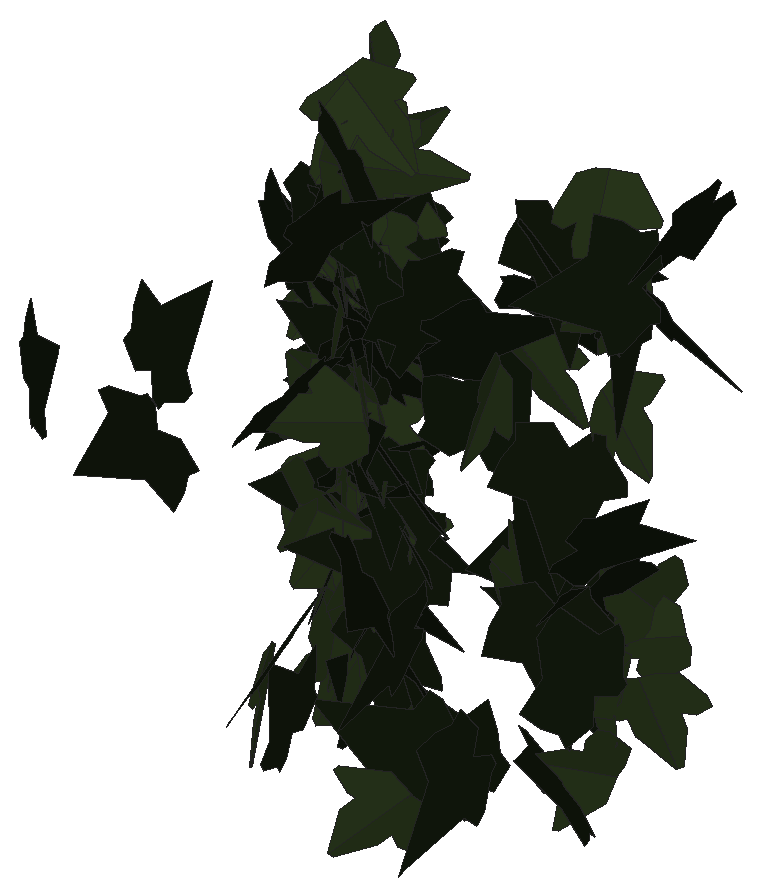
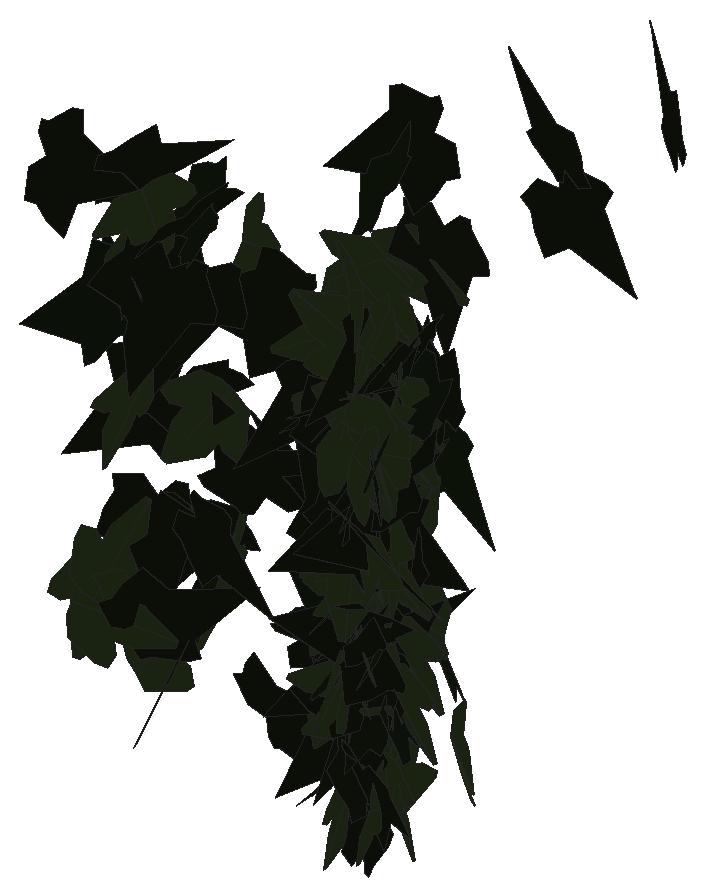
# SketchUp Ruby script. Lengths in inches.
U = 1.inch
M = Sketchup.active_model
def pt(a) = Geom::Point3d.new(a.map { |v| v * U })
def face(e, loops, mat)
  f = e.add_face(loops[0].map { |a| pt(a) })
  loops[1..].each { |l| e.add_face(l.map { |a| pt(a) }).erase! }
  f.material = f.back_material = mat if mat
  f
end
# faces: each face lists its corners as indices into pts; further lists are holes
def faces(e, pts, list, mat = nil) = list.each { |f| face(e, (f[0].is_a?(Array) ? f : [f]).map { |l| l.map { |i| pts[i] } }, mat) }
# xy, xz, yz: faces in a plane at the given z, y or x. An outline is a flat list of corners, or four numbers for a rectangle; further outlines are holes
def ring(l) = l.size == 4 ? [[l[0], l[1]], [l[2], l[1]], [l[2], l[3]], [l[0], l[3]]] : l.each_slice(2).to_a
def flat(e, list, mat, &to3) = list.each { |f| face(e, (f[0].is_a?(Array) ? f : [f]).map { |l| ring(l).map { |u, v| to3.(u, v) } }, mat) }
def xy(e, z, list, mat = nil) = flat(e, list, mat) { |x, y| [x, y, z] }
def xz(e, y, list, mat = nil) = flat(e, list, mat) { |x, z| [x, y, z] }
def yz(e, x, list, mat = nil) = flat(e, list, mat) { |y, z| [x, y, z] }
def lines(e, pts, list) = list.each { |a, b| e.add_line(pt(pts[a]), pt(pts[b])) }
# prism: a flat outline (further loops are holes) pulled along v
def prism(e, loops, v, mat = nil)
  f = face(e, loops, mat); d = Geom::Vector3d.new(v.map { |x| x * U })
  f.pushpull(f.normal.samedirection?(d) ? d.length : -d.length)
end
def box(e, o, s, mat = nil) = prism(e, [[o, [o[0] + s[0], o[1], o[2]], [o[0] + s[0], o[1] + s[1], o[2]], [o[0], o[1] + s[1], o[2]]]], [0, 0, s[2]], mat)
def at(x, y, z, deg = 0) = Geom::Transformation.translation(pt([x, y, z])) * Geom::Transformation.rotation(ORIGIN, Z_AXIS, deg.degrees)
def axes(o, x, y, z) = Geom::Transformation.new([*x, 0, *y, 0, *z, 0, *pt(o).to_a, 1])
def part(name) = M.definitions.add(name)
# library, detail: a bought-in or finely detailed component or shape, given as its bounding box
def library(name, o, s) = part(name).tap { |d| box(d.entities, o, s) }
def detail(e, o, s) = box(e.add_group.entities, o, s)
def put(e, d, t, mat = nil) = e.add_instance(d, t).tap { |i| i.material = mat if mat }
def group(e, t, mat = nil) = e.add_group.tap { |g| g.transformation = t; g.material = mat if mat }.entities
root = M.entities
M.materials.add("efeu1").color = [18, 25, 13]
M.materials.add("efeu2").color = [43, 57, 29]
c1 = part("ivyleaf_10")
p = [[0,0.5,-0.03],[-0.0625,2.02,-0.43],[-0.19,2.01,-0.46],[-0.54,1.05,-0.29],[-0.52,0.625,-0.18],[-0.83,0.76,-0.28],
  [-1.16,0.64,-0.33],[-1.15,0.33,-0.24],[-0.77,-0.39,0.02],[-0.3,-0.51,0.16],[0.04,-0.48,0.23],[-0.02,2.01,-0.4375],
  [-0.06,2.01,-0.43],[0.04,-0.49,0.23],[0.67,-0.49,0.14],[1.38,0.36,-0.2],[1.375,0.51,-0.24],[0.81,0.65,-0.19],
  [0.62,0.59,-0.15],[0.6,1.09,-0.28],[0.5,1.23,-0.31]]
faces(c1.entities,p,[[0,1,2,3,4,5,6,7,8,9,10],[11,12,0,13,14,15,16,17,18,19,20]],"efeu2")
c2 = part("ivyleaf_9")
p = [[1.54,2.16,1.25],[1.36,2.04,1.19],[-0.21,0.99,0.68],[-0.71,1.11,0.82],[-0.85,0.86,0.67],[-0.8,0.17,0.21],
  [-0.9,-0.01,0.1],[-0.67,-0.16,-0.02],[-0.08,-0.08,-0.05],[-0.03,-0.6,-0.4],[0.65,-0.88,-0.66],[0.83,-0.6,-0.49],
  [1.29,-0.42,-0.43],[1.8125,-0.07,-0.26],[1.21,0.44,0.15]]
faces(c2.entities,p,[[0,1,2,3,4,5,6,7,8,9,10,11,12,13,14]],"efeu1")
put(root,c1,axes([46.83,221.1,208.74],[0.39164,-0.18559,-0.24935],[-0.22582,0.10576,-0.43338],[0.2136,0.45208,-0.00098]))
put(root,c1,axes([46.84,221.05,209.32],[0.42383,-0.11987,-0.23664],[-0.22766,0.06455,-0.44046],[0.13615,0.48111,0.00014]))
put(root,c1,axes([46.65,221.74,207.45],[-0.01343,0.23322,-0.44207],[0.03841,-0.44044,-0.23353],[-0.49834,-0.04023,-0.00609]))
put(root,c2,axes([46.47,220.7,212.16],[-0.01841,0.02309,0.49913],[0.23908,-0.43817,0.02909],[0.43875,0.23974,0.00509]))
put(root,c1,axes([46.95,221.2,210.63],[-0.43209,0.10694,0.22774],[-0.22152,0.05288,-0.44512],[-0.11929,-0.48556,0.00168]))
put(root,c1,axes([46.85,221.12,210.37],[-0.18313,-0.32588,-0.33206],[-0.16064,-0.29062,0.37381],[-0.43664,0.2436,0.00175]))
put(root,c2,axes([46.55,221.15,212.125],[0.41245,-0.22857,-0.16625],[0.14512,-0.08112,0.47155],[-0.24254,-0.43723,-0.00058]))
put(root,c2,axes([46.96,221.4,209.11],[-0.12755,-0.05771,0.48],[-0.33346,-0.34894,-0.13056],[0.35006,-0.35342,0.05052]))
put(root,c2,axes([47.17,221.42,210.67],[-0.37965,0.24229,0.21716],[-0.1893,0.10694,-0.45025],[-0.26464,-0.4241,0.01053]))
put(root,c2,axes([46.76,221.76,207.88],[-0.37467,-0.03207,-0.32954],[0.32765,0.03568,-0.376],[0.04763,-0.49769,-0.00572]))
put(root,c1,axes([47.1,221.13,210.36],[0.25748,-0.10183,-0.41633],[-0.38457,0.15956,-0.27686],[0.18924,0.46279,0.00384]))
put(root,c1,axes([46.7,220.12,207.51],[0.27486,-0.30783,0.28229],[0.20205,-0.19776,-0.41239],[0.36555,0.34078,0.01568]))
put(root,c1,axes([46.9375,221.21,211.97],[0.34959,0.23007,-0.2736],[-0.22223,-0.15987,-0.41839],[-0.28,0.41414,-0.00952]))
put(root,c1,axes([46.78,221.73,211.82],[0.06072,-0.36268,0.33878],[0.13761,-0.31562,-0.36255],[0.47684,0.13727,0.06148]))
put(root,c1,axes([47.01,221.65,212],[-0.2421,-0.38149,0.21413],[-0.11452,-0.18094,-0.45183],[0.42222,-0.26782,0.00024]))
put(root,c2,axes([47.05,221.33,210.73],[-0.03029,0.09287,-0.49036],[-0.03619,-0.49038,-0.09064],[-0.49777,0.03,0.03643]))
put(root,c1,axes([47.05,221.375,212.01],[0.1141,0.18818,-0.44896],[-0.30826,-0.32897,-0.21623],[-0.37677,0.32614,0.04095]))
put(root,c2,axes([46.73,221.04,208.12],[-0.0222,0.36747,0.33834],[0.0225,-0.3376,0.36813],[0.499,0.03157,-0.00155]))
put(root,c1,axes([46.91,221.14,207.38],[-0.14529,-0.42532,-0.21908],[-0.06763,-0.2084,0.44944],[-0.47362,0.16023,0.00303]))
put(root,c2,axes([46.77,220.98,212.99],[0.21687,-0.37209,-0.254],[-0.12227,0.22271,-0.43064],[0.43361,0.2489,0.0056]))
put(root,c1,axes([47.07,221.3,207.84],[0.43528,-0.02059,0.24517],[-0.24488,0.01199,0.43576],[-0.02383,-0.49943,0.00035]))
put(root,c1,axes([47.01,220.91,213.27],[-0.10849,0.25279,0.41752],[-0.14944,0.38997,-0.27494],[-0.46465,-0.18445,-0.00906]))
put(root,c2,axes([46.9,221.2,210.39],[0.32605,-0.2109,-0.31498],[-0.26823,0.1652,-0.38828],[0.26785,0.42217,-0.00541]))
put(root,c2,axes([46.79,221.75,211.54],[0.28591,-0.31711,-0.26019],[0.22914,-0.13959,0.42191],[-0.34022,-0.36049,0.06551]))
put(root,c1,axes([47.06,221.625,210.54],[-0.48962,-0.09666,0.03043],[-0.02974,-0.00648,-0.49907],[0.09687,-0.49053,0.00059]))
put(root,c2,axes([46.86,221.09,210.72],[0.14251,0.18608,0.44166],[0.26871,0.35051,-0.23439],[-0.39684,0.30417,-0.0001]))
put(root,c2,axes([47,221.09,213.14],[0.00356,0.06584,-0.49563],[-0.22599,0.44234,0.05714],[0.446,0.22361,0.03291]))
put(root,c2,axes([47.23,221.41,210.78],[0.02764,0.05595,0.49609],[-0.45174,-0.20871,0.04871],[0.21253,-0.4509,0.03901]))
put(root,c1,axes([47.12,221.26,213.85],[0.38338,0.21117,-0.24171],[-0.21503,-0.11056,-0.43765],[-0.23829,0.43953,0.00605]))
put(root,c1,axes([46.91,221.25,211.77],[0.22561,-0.33797,0.29134],[0.18754,-0.22441,-0.40555],[0.40488,0.29227,0.02551]))
put(root,c1,axes([46.84,221.83,214.12],[-0.21314,0.15217,-0.42593],[0.23213,-0.3673,-0.24739],[-0.38818,-0.3032,0.08593]))
put(root,c1,axes([47.17,220.85,207.33],[0.35129,-0.2722,-0.22912],[-0.17286,0.15085,-0.44425],[0.31098,0.39134,0.01188]))
put(root,c1,axes([46.68,221.39,211.86],[0.03035,-0.0241,0.4985],[0.45238,0.21225,-0.01728],[-0.21078,0.45207,0.03469]))
put(root,c1,axes([47.03,221,212.39],[-0.04,0.29848,0.39913],[-0.04623,0.39647,-0.30112],[-0.49625,-0.061,-0.00412]))
put(root,c1,axes([46.92,221.02,212.55],[-0.20701,0.34767,-0.29373],[0.14175,-0.25739,-0.40455],[-0.4325,-0.25076,0.008]))
put(root,c2,axes([47.01,221.44,206.71],[0.03763,0.09783,0.48889],[-0.16723,-0.4594,0.1048],[0.4697,-0.1714,-0.00186]))
put(root,c1,axes([47.05,220.77,209.29],[-0.23254,-0.38717,-0.21454],[0.10721,0.18586,-0.45162],[0.42945,-0.25604,-0.00342]))
put(root,c2,axes([47.22,221.61,209.625],[-0.45645,-0.20252,0.0253],[-0.01998,-0.01732,-0.4993],[0.20311,-0.45682,0.00772]))
put(root,c2,axes([46.95,221.32,208.6],[0.4608,-0.05926,-0.18479],[-0.18126,0.03862,-0.46438],[0.06931,0.49497,0.01411]))
put(root,c2,axes([46.68,221.06,211.44],[0.34659,-0.16227,0.32178],[0.29807,-0.12185,-0.3825],[0.20256,0.45697,0.01227]))
put(root,c2,axes([47.23,221.55,211.9375],[0.17385,0.06608,0.46412],[-0.43069,-0.17299,0.18596],[0.18515,-0.46444,-0.00323]))
put(root,c2,axes([46.9,221.16,209.29],[0.08639,0.40443,-0.28102],[0.03407,0.27972,0.41303],[0.4913,-0.09051,0.02078]))
put(root,c2,axes([46.9,221.53,211.93],[-0.14439,-0.01708,-0.47839],[0.47401,-0.07488,-0.1404],[-0.06685,-0.49407,0.03781]))
put(root,c1,axes([46.76,220.57,209.26],[-0.0606,-0.04962,0.49383],[0.48949,0.07625,0.06773],[-0.08203,0.49165,0.03934]))
put(root,c1,axes([46.97,220.99,212.16],[0.40596,0.19019,-0.22142],[0.19999,0.09504,0.4483],[0.21261,-0.45254,0.00109]))
put(root,c1,axes([46.96,221.26,210.3],[0.16139,-0.1948,0.43128],[0.28356,-0.32501,-0.25291],[0.37888,0.32622,0.00557]))
put(root,c1,axes([47.08,221.08,209.82],[-0.08278,0.41112,-0.27227],[0.05389,-0.26688,-0.41937],[-0.49015,-0.09877,-0.00012]))
put(root,c2,axes([47.02,221.43,207.48],[0.03972,0.38769,0.31324],[-0.03437,-0.31136,0.38971],[0.49723,-0.05249,0.00192]))
put(root,c2,axes([47.02,221.23,210.73],[0.23471,0.22948,0.37716],[0.23848,0.29357,-0.32703],[-0.37154,0.3334,0.02836]))
put(root,c1,axes([47.17,221.42,208.38],[0.18777,0.43607,-0.15681],[0.06091,0.1445,0.47477],[0.45938,-0.1974,0.00114]))
put(root,c1,axes([47.07,221.65,212.46],[0.46651,0.15649,0.08876],[0.08424,0.02797,-0.49206],[-0.15897,0.47406,-0.00027]))
put(root,c1,axes([47.24,221.2,208.53],[0.00994,-0.49164,-0.09049],[0.04746,0.09103,-0.48935],[0.49764,0.00114,0.04848]))
put(root,c2,axes([46.9375,220.9375,209.95],[-0.02063,-0.03444,0.49839],[0.31276,-0.38985,-0.01399],[0.38956,0.31117,0.03763]))
put(root,c1,axes([47.03,221.47,213.14],[-0.15521,-0.34336,0.32865],[0.25572,0.2311,0.36221],[-0.40064,0.28053,0.10387]))
put(root,c2,axes([46.99,221.22,208.97],[0.02468,0.01091,-0.49927],[0.19457,0.46017,0.01967],[0.45993,-0.19525,0.01847]))
put(root,c1,axes([47.125,221.33,210],[0.15504,0.37581,0.29109],[0.09136,0.27692,-0.40617],[-0.46649,0.17913,0.0172]))
put(root,c2,axes([47.05,221.28,208.54],[0.42244,0.25339,0.08564],[-0.07422,-0.04275,0.49261],[0.25697,-0.42891,0.00149]))
put(root,c2,axes([47.22,221.48,208.72],[0.28897,-0.4002,-0.07961],[0.0523,-0.06042,0.49357],[-0.40467,-0.29359,0.00694]))
put(root,c1,axes([47.2,221.41,207.41],[0.03675,-0.47593,-0.14878],[0.1631,0.15245,-0.44739],[0.47122,-0.01565,0.16645]))
put(root,c1,axes([47.23,221.53,208.93],[-0.04885,0.42067,-0.2658],[0.03775,-0.26318,-0.42345],[-0.49617,-0.06143,-0.00605]))
put(root,c1,axes([47.08,221.27,208.9],[0.23776,-0.27731,-0.34142],[0.22173,-0.25962,0.36528],[-0.37987,-0.32511,-0.00048]))
put(root,c1,axes([46.96,221.17,209.26],[0.07199,-0.00591,0.49475],[0.49319,0.04106,-0.07127],[-0.03979,0.49828,0.01174]))
put(root,c2,axes([47.16,221.1875,208.3],[0.48473,0.11647,0.0384],[0.03679,0.01125,-0.49852],[-0.11698,0.48612,0.00233]))
put(root,c1,axes([47.1875,221.44,208.75],[0.3142,0.32981,0.20616],[0.13789,0.15336,-0.45549],[-0.36368,0.34308,0.00542]))
put(root,c2,axes([47.1,221.22,209.75],[0.3366,-0.17318,-0.32667],[0.29516,-0.14018,0.37845],[-0.22267,-0.44761,0.00786]))
put(root,c1,axes([47.08,221.14,214.03],[0.30949,0.16973,0.35413],[0.3178,0.15662,-0.3528],[-0.23069,0.44347,-0.01093]))
put(root,c2,axes([47.02,221.27,210.87],[0.25708,-0.1956,0.38165],[0.33213,-0.19069,-0.32145],[0.2713,0.41878,0.03188]))
put(root,c2,axes([47.13,221.51,212.46],[0.13927,-0.44393,-0.18312],[0.17556,0.22453,-0.41081],[0.44697,0.05013,0.21842]))
put(root,c2,axes([47.26,221.4,209.82],[0.04725,-0.4851,0.11157],[0.05297,-0.10653,-0.48564],[0.49494,0.05771,0.04132]))
put(root,c2,axes([47.26,215.53,213.09],[-0.03796,0.13422,0.48015],[0.14176,-0.45876,0.13945],[0.47798,0.14672,-0.00323]))
put(root,c2,axes([47.11,221.63,211.11],[0.42681,0.01465,-0.26003],[0.25955,0.01748,0.427],[0.0216,-0.49948,0.00732]))
put(root,c1,axes([47.2,221.32,208.38],[0.21013,-0.16588,-0.42229],[0.32391,-0.27102,0.26764],[-0.31769,-0.38604,-0.00644]))
put(root,c1,axes([47.25,221.22,213.23],[-0.12385,-0.06867,-0.47953],[0.40146,0.26244,-0.14127],[0.27109,-0.42001,-0.00988]))
put(root,c2,axes([47.31,221.3125,212.26],[0.04712,-0.48,0.13182],[0.0535,-0.12676,-0.4807],[0.49489,0.0594,0.03942]))
put(root,c1,axes([47.21,221.34,212.23],[-0.19398,0.06559,-0.45614],[0.43333,-0.14247,-0.20477],[-0.15684,-0.47476,-0.00157]))
put(root,c2,axes([47.34,221.46,207.5625],[-0.02149,-0.46574,0.18062],[0.09194,-0.18139,-0.45678],[0.49101,0.01358,0.09343]))
put(root,c2,axes([47.22,221.55,209.2],[0.20636,-0.35399,0.28654],[0.14295,-0.24834,-0.40975],[0.43241,0.25103,-0.00129]))
put(root,c1,axes([47.83,220.3125,210.88],[0.05314,-0.03429,-0.49598],[-0.2254,0.44294,-0.05477],[0.44314,0.22941,0.03162]))
put(root,c2,axes([47.27,221.4,209.59],[0.21745,-0.26691,0.36259],[0.23823,-0.27347,-0.34418],[0.38205,0.32244,0.00824]))
put(root,c2,axes([48,221.1,208.9375],[-0.14158,-0.27391,-0.39361],[-0.14337,-0.36746,0.30728],[-0.4576,0.19987,0.02551]))
put(root,c2,axes([48.11,218.79,207.86],[-0.11697,0.26939,0.40466],[-0.15179,0.37516,-0.29362],[-0.46182,-0.19154,-0.00598]))
put(root,c2,axes([48.21,216.38,212.49],[0.06849,0.07329,-0.48983],[-0.41416,-0.26272,-0.09722],[-0.27163,0.41905,0.02472]))
put(root,c2,axes([47.6875,220.98,207.73],[0.31046,-0.07247,-0.38518],[0.38347,-0.0454,0.31763],[-0.08101,-0.49263,0.02739]))
put(root,c2,axes([48.03,220.82,212.08],[0.05174,-0.02094,-0.49688],[-0.11564,0.48536,-0.03249],[0.48368,0.11828,0.04538]))
put(root,c2,axes([47.98,216.67,213.08],[-0.18121,0.22955,0.40555],[0.24409,-0.32391,0.2924],[0.39697,0.30396,0.00533]))
put(root,c2,axes([47.91,219.98,214.15],[0.15381,-0.35684,0.31466],[0.1188,-0.29141,-0.38855],[0.46068,0.19429,-0.00486]))
put(root,c2,axes([48.75,217.85,212.45],[-0.03205,0.4973,0.04081],[-0.00766,0.0404,-0.49831],[-0.49891,-0.03256,0.00503]))
put(root,c2,axes([48.54,218.36,214],[-0.03569,0.30625,-0.39362],[-0.0757,0.38673,0.30775],[0.49295,0.08156,0.01876]))
put(root,c2,axes([48.92,217.76,209.69],[-0.3057,0.35989,-0.1644],[0.09716,-0.13311,-0.47206],[-0.38354,-0.32057,0.01145]))
put(root,c1,axes([49.17,218.34,212.1],[-0.09672,-0.01649,0.49028],[-0.43873,-0.22064,-0.09397],[0.21945,-0.44838,0.02821]))
put(root,c2,axes([48.73,221.1,210.52],[-0.30496,-0.01576,0.39592],[0.39095,-0.09328,0.29742],[0.06449,0.49097,0.06921]))
put(root,c2,axes([49.33,220.26,207.04],[-0.02787,0.0692,0.4944],[-0.35442,0.34598,-0.06841],[-0.35158,-0.35427,0.02977]))
put(root,c1,axes([49.38,218.95,207.34],[-0.28795,-0.18645,0.36376],[-0.2909,-0.21912,-0.34258],[0.28716,-0.40893,0.01772]))
put(root,c2,axes([49.48,219.4375,207.63],[-0.31003,-0.2799,-0.27484],[-0.20246,-0.18589,0.41768],[-0.336,0.37027,0.00192]))
put(root,c1,axes([49.19,221.39,211.62],[-0.42587,0.00383,-0.26195],[0.26197,0.00051,-0.42588],[-0.00299,-0.49999,-0.00244]))
put(root,c2,axes([49.54,218.18,210.47],[0.2309,0.03902,-0.44177],[-0.44015,-0.04087,-0.23366],[-0.05434,0.4968,0.01548]))
put(root,c2,axes([49.15,220.07,212.3],[0.15272,0.30223,-0.36787],[0.13375,0.34355,0.33777],[0.45693,-0.20157,0.02409]))
put(root,c2,axes([49.84,220.9,209.65],[-0.0179,-0.01902,-0.49932],[-0.47062,-0.16726,0.02324],[-0.16792,0.47081,-0.01191]))
put(root,c2,axes([49.7,218.79,209.58],[-0.41485,0.22749,-0.1617],[0.13398,-0.0918,-0.47289],[-0.24484,-0.43568,0.01521]))
put(root,c1,axes([49.51,220.79,209.125],[-0.2045,0.31087,0.33397],[0.1891,-0.27532,0.37207],[0.41524,0.27848,-0.00497]))
put(root,c2,axes([50.18,221.47,208.41],[-0.07335,0.00571,0.49456],[-0.49267,-0.04486,-0.07256],[0.04354,-0.49795,0.01221]))
put(root,c2,axes([49.82,220.85,212.85],[0.37362,0.32103,-0.08571],[-0.06577,-0.05497,-0.4926],[-0.3257,0.37936,0.00116]))
put(root,c2,axes([49.77,221.14,208.3],[0.31992,-0.23144,-0.30674],[-0.23831,0.19359,-0.39462],[0.30143,0.39869,0.01356]))
put(root,c2,axes([50,221.24,212.96],[0.3324,0.35997,-0.09965],[-0.06706,-0.07371,-0.48997],[-0.36744,0.3391,-0.00073]))
put(root,c2,axes([50.01,220.92,213.53],[0.00891,-0.49899,-0.03043],[0.00711,0.03056,-0.49901],[0.49987,0.00846,0.00764]))
put(root,c2,axes([49.96,220.59,213.53],[0.41912,-0.27226,0.01463],[0.01244,-0.00771,-0.49979],[0.27237,0.4193,0.00031]))
put(root,c1,axes([50.24,221.34,213.87],[0.25006,0.4062,-0.14991],[-0.07723,-0.1285,-0.477],[-0.42604,0.26171,-0.00152]))
put(root,c1,axes([50.69,221.76,208.58],[-0.09252,-0.04608,0.4892],[-0.39731,-0.28588,-0.10207],[0.28912,-0.40761,0.01629]))
put(root,c1,axes([50.33,219.42,212.46],[-0.0628,0.28107,-0.40872],[-0.00971,-0.4126,-0.28225],[-0.49594,-0.02752,0.05728]))
put(root,c2,axes([50.34,220.59,211.13],[-0.17179,-0.45133,-0.12958],[0.03357,0.12583,-0.48274],[0.46836,-0.17456,-0.01293]))
put(root,c1,axes([50.4,221.3,211.38],[-0.02325,0.45597,0.20385],[-0.02546,0.20272,-0.45635],[-0.49881,-0.0316,0.01379]))
put(root,c2,axes([50.59,220.69,209.57],[0.03035,0.49415,-0.06997],[-0.00707,-0.06967,-0.49507],[-0.49903,0.03104,0.00275]))
put(root,c2,axes([50.36,220.35,209.38],[-0.25586,-0.30475,-0.30275],[0.20387,0.22403,-0.3978],[0.37812,-0.32701,0.00962]))
put(root,c1,axes([50.64,221.625,208.98],[-0.15812,-0.31439,-0.35518],[-0.1581,-0.31806,0.35192],[-0.44722,0.2236,0.00117]))
put(root,c1,axes([50.78,220.57,207.47],[-0.14279,-0.1433,-0.45725],[-0.28149,-0.36103,0.20105],[-0.38778,0.31484,0.02243]))
put(root,c1,axes([50.63,221.27,212.81],[-0.02611,0.05585,0.49618],[0.06258,-0.49258,0.05874],[0.49538,0.06517,0.01874]))
put(root,c1,axes([50.46,221.06,208.18],[0.21846,-0.27404,-0.35662],[0.24123,-0.26321,0.35004],[-0.37958,-0.325,0.01721]))
put(root,c2,axes([50.64,221.25,212.79],[-0.30356,0.00538,-0.39727],[0.39679,-0.02143,-0.30348],[-0.02029,-0.49951,0.00874]))
put(root,c2,axes([50.68,220.06,207.53],[0.3529,-0.33761,-0.10714],[0.07842,-0.07302,0.48838],[-0.34541,-0.36151,0.00141]))
put(root,c2,axes([51.17,219.95,208.86],[-0.44697,-0.04554,-0.21941],[-0.2182,-0.023,0.44929],[-0.05102,0.49739,0.00069]))
put(root,c2,axes([50.48,221.63,212.58],[0.41229,-0.20154,0.1985],[0.17828,-0.08729,-0.45891],[0.21963,0.44918,-0.00012]))
put(root,c2,axes([51.28,220.57,213.46],[-0.22004,-0.14203,0.42592],[-0.32364,-0.27857,-0.2601],[0.31119,-0.39016,0.03066]))
put(root,c2,axes([51.22,217.86,208.98],[-0.47241,0.0363,-0.15973],[0.15793,-0.02847,-0.47355],[-0.04347,-0.49787,0.01543]))
put(root,c2,axes([51.03,219.98,210.51],[0.26081,0.28253,0.31961],[0.2204,0.23149,-0.38449],[-0.36524,0.34145,-0.00379]))
put(root,c1,axes([51.19,220.87,208.46],[-0.43302,-0.21865,-0.1212],[0.11352,0.04399,-0.48495],[0.22274,-0.4475,0.01155]))
put(root,c2,axes([51.47,221.53,214.0625],[-0.23759,0.04709,-0.43742],[0.22286,-0.41574,-0.16581],[-0.37932,-0.27375,0.17656]))
